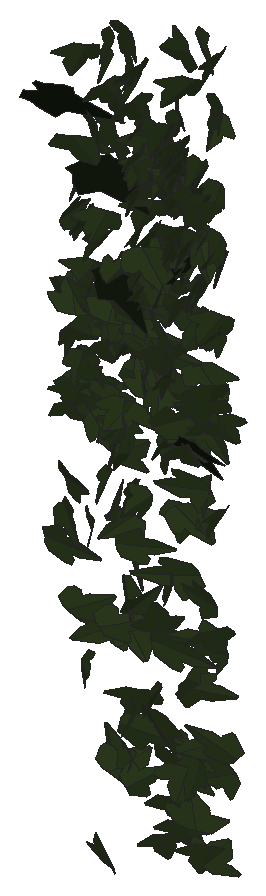
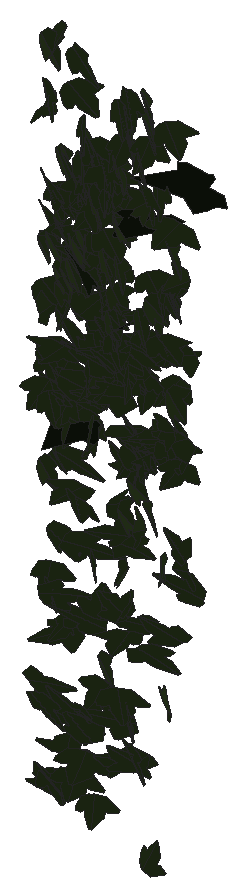
# SketchUp Ruby script. Lengths in millimetres.
U = 1.mm
M = Sketchup.active_model
def pt(a) = Geom::Point3d.new(a.map { |v| v * U })
def face(e, loops, mat)
  f = e.add_face(loops[0].map { |a| pt(a) })
  loops[1..].each { |l| e.add_face(l.map { |a| pt(a) }).erase! }
  f.material = f.back_material = mat if mat
  f
end
# faces: each face lists its corners as indices into pts; further lists are holes
def faces(e, pts, list, mat = nil) = list.each { |f| face(e, (f[0].is_a?(Array) ? f : [f]).map { |l| l.map { |i| pts[i] } }, mat) }
# xy, xz, yz: faces in a plane at the given z, y or x. An outline is a flat list of corners, or four numbers for a rectangle; further outlines are holes
def ring(l) = l.size == 4 ? [[l[0], l[1]], [l[2], l[1]], [l[2], l[3]], [l[0], l[3]]] : l.each_slice(2).to_a
def flat(e, list, mat, &to3) = list.each { |f| face(e, (f[0].is_a?(Array) ? f : [f]).map { |l| ring(l).map { |u, v| to3.(u, v) } }, mat) }
def xy(e, z, list, mat = nil) = flat(e, list, mat) { |x, y| [x, y, z] }
def xz(e, y, list, mat = nil) = flat(e, list, mat) { |x, z| [x, y, z] }
def yz(e, x, list, mat = nil) = flat(e, list, mat) { |y, z| [x, y, z] }
def lines(e, pts, list) = list.each { |a, b| e.add_line(pt(pts[a]), pt(pts[b])) }
# prism: a flat outline (further loops are holes) pulled along v
def prism(e, loops, v, mat = nil)
  f = face(e, loops, mat); d = Geom::Vector3d.new(v.map { |x| x * U })
  f.pushpull(f.normal.samedirection?(d) ? d.length : -d.length)
end
def box(e, o, s, mat = nil) = prism(e, [[o, [o[0] + s[0], o[1], o[2]], [o[0] + s[0], o[1] + s[1], o[2]], [o[0], o[1] + s[1], o[2]]]], [0, 0, s[2]], mat)
def at(x, y, z, deg = 0) = Geom::Transformation.translation(pt([x, y, z])) * Geom::Transformation.rotation(ORIGIN, Z_AXIS, deg.degrees)
def axes(o, x, y, z) = Geom::Transformation.new([*x, 0, *y, 0, *z, 0, *pt(o).to_a, 1])
def part(name) = M.definitions.add(name)
# library, detail: a bought-in or finely detailed component or shape, given as its bounding box
def library(name, o, s) = part(name).tap { |d| box(d.entities, o, s) }
def detail(e, o, s) = box(e.add_group.entities, o, s)
def put(e, d, t, mat = nil) = e.add_instance(d, t).tap { |i| i.material = mat if mat }
def group(e, t, mat = nil) = e.add_group.tap { |g| g.transformation = t; g.material = mat if mat }.entities
root = M.entities
M.materials.add("efeu1").color = [18, 25, 13]
M.materials.add("efeu2").color = [43, 57, 29]
c1 = part("ivyleaf_10")
p = [[0,12.8,-0.8],[-1.5,51.3,-10.9],[-4.9,51,-11.6],[-13.6,26.5,-7.3],[-13.2,15.9,-4.6],[-21.1,19.3,-7.2],
  [-29.5,16.3,-8.3],[-29.2,8.3,-6.2],[-19.7,-9.8,0.5],[-7.6,-13,4],[1,-12.2,5.8],[-0.4,51.1,-11.1],
  [-1.5,51.1,-10.9],[1,-12.4,5.9],[16.9,-12.4,3.5],[35.1,9.1,-5.1],[35,12.9,-6.1],[20.5,16.4,-4.9],
  [15.8,15,-3.8],[15.3,27.6,-7.1],[12.8,31.3,-7.8]]
faces(c1.entities,p,[[0,1,2,3,4,5,6,7,8,9,10],[11,12,0,13,14,15,16,17,18,19,20]],"efeu2")
c2 = part("ivyleaf_9")
p = [[39.1,54.8,31.7],[34.5,51.8,30.2],[-5.3,25.2,17.3],[-17.9,28.3,20.9],[-21.6,21.7,17],[-20.2,4.3,5.3],
  [-22.9,-0.3,2.5],[-17.1,-4,-0.6],[-2,-2.1,-1.2],[-0.7,-15.4,-10.1],[16.6,-22.3,-16.7],[21.1,-15.1,-12.5],
  [32.7,-10.7,-11],[46.1,-1.8,-6.6],[30.8,11.2,3.8]]
faces(c2.entities,p,[[0,1,2,3,4,5,6,7,8,9,10,11,12,13,14]],"efeu1")
put(root,c1,axes([1270.6,1047.9,459],[-0.48285,0.07092,0.58722],[0.98278,-0.28506,0.25752],[0.54901,0.57266,0.05547]))
put(root,c2,axes([1259.8,1017.1,959.8],[0.35127,0.22644,-0.71654],[0.93732,0.52083,0.29145],[1.08021,-0.52557,-0.01989]))
put(root,c1,axes([1290.7,1041.6,666],[0.08143,-0.71118,0.27788],[0.14243,-0.27307,-0.7104],[1.44618,0.06694,0.05432]))
put(root,c1,axes([1286.2,1033.5,567.7],[-0.64923,-0.40429,-0.35378],[0.45804,0.25966,-0.5288],[0.91411,-0.41725,0.01371]))
put(root,c1,axes([1293.5,1040.9,809.3],[0.45294,-0.6195,-0.05972],[-0.02572,0.05878,-0.66359],[1.18422,0.23822,0.00843]))
put(root,c1,axes([1274.2,1035.2,428.7],[0.55128,-0.2534,0.61949],[0.97945,-0.34727,-0.38268],[0.81446,0.58913,0.04089]))
put(root,c1,axes([1299.5,1033.3,593.1],[-0.71097,-0.53152,0.10227],[-0.08643,-0.09305,-0.64947],[1.02652,-0.37597,0.01615]))
put(root,c1,axes([1295.2,1017.3,814.9],[0.19746,-0.12143,0.71883],[-0.29901,0.70528,0.14182],[-1.35485,-0.17335,0.07346]))
put(root,c1,axes([1303.5,1047.5,741.8],[-0.68919,-0.44252,0.31408],[-0.16618,-0.32515,-0.5588],[1.01932,-0.35221,0.12126]))
put(root,c1,axes([1271.1,1024.5,393.3],[-0.1705,-0.0206,0.6802],[1.29073,0.0539,0.09095],[-0.10685,0.68395,0.01332]))
put(root,c1,axes([1299.9,1041.3,809.1],[-0.14305,-0.63344,0.13711],[0.05173,-0.14099,-0.63646],[1.2324,-0.06761,0.04263]))
put(root,c1,axes([1292.6,1037,900.1],[-1.1968,-0.1578,-0.2539],[0.4826,0.03165,-0.64769],[0.30134,-0.67742,0.02889]))
put(root,c1,axes([1284.1,1024.8,721.7],[-0.79131,0.25289,-0.44889],[0.7383,-0.22596,-0.4866],[-0.64532,-0.56861,-0.00627]))
put(root,c1,axes([1300.7,1039.6,807.5],[-0.06985,-0.5542,-0.34902],[0.10152,0.34587,-0.55481],[1.24234,-0.05942,0.02571]))
put(root,c1,axes([1301.3,1017.7,704.4],[0.54287,0.60614,-0.14799],[0.04541,0.152,0.66858],[1.18663,-0.28312,0.04212]))
put(root,c1,axes([1303.2,1029.4,864.3],[0.39037,-0.67223,-0.01479],[0.00033,0.01552,-0.70281],[1.27971,0.20506,0.0047]))
put(root,c1,axes([1307.4,1027.7,1026.5],[-0.56433,-0.63131,0.13286],[-0.04648,-0.13513,-0.69661],[1.22695,-0.29549,0.03472]))
put(root,c1,axes([1291.5,1051,624.8],[-0.50661,0.32371,-0.48857],[0.53245,-0.40133,-0.41833],[-0.98013,-0.38534,0.02527]))
put(root,c1,axes([1298.9,1022.8,673.5],[-0.4007,-0.39208,-0.52059],[0.46515,0.45965,-0.44503],[1.14983,-0.32258,-0.00138]))
put(root,c1,axes([1295,1047.7,236.8],[-0.08005,-0.11947,-0.66552],[0.28496,-0.65189,0.10756],[-1.25491,-0.14041,0.06688]))
put(root,c1,axes([1299.5,1029.8,632.5],[0.81136,-0.41907,0.26503],[0.33228,-0.20028,-0.5975],[0.88325,0.4603,-0.01868]))
put(root,c1,axes([1290.9,1031.7,601.4],[-0.59807,-0.21352,-0.5687],[0.98704,0.23908,-0.37634],[0.60197,-0.60416,0.05206]))
put(root,c1,axes([1314.7,1030.7,423.7],[0.18319,-0.2164,-0.62084],[-0.10033,0.6229,-0.22529],[1.24728,0.08189,0.07306]))
put(root,c1,axes([1320.1,1045.9,787.2],[0.01443,-0.57265,0.3385],[0.01646,-0.3384,-0.57269],[1.26592,0.01093,0.00359]))
put(root,c1,axes([1302.7,1034.1,604.2],[0.18724,0.03395,0.63404],[0.5869,0.55831,-0.07774],[-1.05635,0.3162,0.06919]))
put(root,c1,axes([1316.3,1036,745.6],[0.49908,-0.57185,0.15686],[0.16781,-0.132,-0.62863],[1.11599,0.27558,0.02438]))
put(root,c1,axes([1333.4,1041.6,299.4],[0.86718,0.14801,-0.46596],[-0.84348,-0.14387,-0.47908],[-0.39283,0.63563,0.00007]))
put(root,c1,axes([1301.9,1024.3,321.7],[0.70088,0.10938,-0.51488],[0.94066,0.14429,0.38416],[0.34459,-0.61636,-0.00144]))
put(root,c1,axes([1324.7,1024.3,937.2],[0.74216,-0.4563,-0.37185],[-0.02289,0.43978,-0.55226],[1.12004,0.31134,0.23511]))
put(root,c1,axes([1328.1,1037.8,817.7],[-0.67576,-0.50671,0.22798],[0.00591,-0.27236,-0.60051],[1.05748,-0.32228,0.14905]))
put(root,c1,axes([1332.1,1038.9,3.3],[-0.90347,0.42743,-0.05893],[-0.08592,0.03792,0.63878],[0.81667,0.47685,0.00202]))
put(root,c1,axes([1335.7,1038.1,933.8],[0.78445,-0.49191,-0.26423],[-0.13252,0.28057,-0.63096],[1.05442,0.40123,0.11728]))
put(root,c1,axes([1327.7,1027.1,564.8],[0.22158,0.70117,0.19962],[0.06315,0.19685,-0.71077],[-1.38606,0.12106,-0.00047]))
put(root,c1,axes([1313,1038.7,590.9],[-0.53445,0.01322,-0.60596],[1.11303,-0.16953,-0.27472],[-0.30303,-0.646,0.05969]))
put(root,c1,axes([1333.1,1036.7,492.4],[0.54302,-0.59955,0.11204],[0.12132,-0.0937,-0.66376],[1.15445,0.29185,0.01705]))
put(root,c1,axes([1337.1,1033,662.6],[-0.46875,-0.56282,-0.21689],[0.1793,0.19551,-0.61431],[1.13386,-0.26359,0.00747]))
put(root,c1,axes([1340,1042.7,762.2],[-0.02894,-0.64209,-0.11858],[0.02389,0.11831,-0.6422],[1.24247,-0.01723,0.00959]))
put(root,c1,axes([1342,1028.2,1025],[0.4556,-0.66517,-0.10263],[-0.02225,0.10481,-0.70652],[1.28073,0.23844,0.02423]))
put(root,c1,axes([1348.5,1037,139.2],[0.92508,-0.27392,0.41375],[-0.68435,0.20469,0.55794],[-0.65079,-0.60461,0.00143]))
put(root,c1,axes([1355.8,1029.8,976.4],[-0.40267,0.41784,0.51326],[-0.80618,0.32854,-0.44207],[-0.96783,-0.44751,0.15469]))
put(root,c1,axes([1328.5,1039.1,679.8],[0.92068,-0.23299,0.34543],[0.6499,-0.08161,-0.53325],[0.4544,0.5888,0.06278]))
put(root,c1,axes([1341.2,1025.6,991.9],[-0.51206,-0.54368,-0.37865],[0.32502,0.33796,-0.60661],[1.21834,-0.31866,0.00268]))
put(root,c1,axes([1349.8,1030.1,457.8],[0.27821,-0.30767,0.66519],[-0.57251,0.59334,0.34054],[-1.27194,-0.33436,-0.00778]))
put(root,c1,axes([1347.6,1023.2,1052.2],[0.49675,-0.66081,-0.1576],[-0.04579,0.15973,-0.70961],[1.29212,0.25971,0.03544]))
put(root,c1,axes([1344.2,1051.1,532.2],[0.27646,-0.54386,0.4039],[0.18386,-0.39222,-0.56288],[1.27611,0.17433,-0.0064]))
put(root,c1,axes([1319.7,1031.1,713.1],[-0.02383,-0.01891,0.72738],[1.38011,-0.0603,0.01092],[0.11416,0.72499,0.01988]))
put(root,c1,axes([1347,1038.5,541.5],[0.18033,-0.49313,-0.41549],[0.15147,0.42569,-0.48708],[1.21787,0.02008,0.1221]))
put(root,c1,axes([1357.9,1037.8,567.6],[-0.40893,-0.47748,0.38443],[-0.28507,-0.35412,-0.52355],[1.13131,-0.26182,0.00703]))
put(root,c1,axes([1340.2,1039.8,918.9],[-0.69761,0.44971,-0.37639],[0.40815,-0.31033,-0.57963],[-1.03881,-0.42393,0.02503]))
put(root,c1,axes([1357.1,1046.1,440.6],[0.52032,0.33514,-0.47041],[-0.63122,-0.335,-0.43142],[-0.89996,0.42872,0.03062]))
put(root,c1,axes([1360.2,1035.4,146.4],[0.39469,-0.40776,-0.52662],[-0.45604,0.46895,-0.45747],[1.18272,0.3169,-0.00065]))
put(root,c1,axes([1347.8,1024.9,754.1],[0.12771,0.21097,-0.64366],[0.39072,0.61005,0.22136],[1.2285,-0.21596,-0.00349]))
put(root,c2,axes([1338.3,1018.8,891.4],[-0.11232,-0.38165,-0.68878],[0.28644,0.67252,-0.38553],[1.47105,-0.16009,0.02248]))
put(root,c1,axes([1348.4,1023.2,708.4],[0.66981,0.50858,-0.26519],[0.29588,0.2149,0.61845],[1.05074,-0.38471,-0.0051]))
put(root,c1,axes([1354,1033.9,567.3],[0.72092,-0.5372,0.01208],[0.00676,-0.01227,-0.65731],[1.02264,0.37879,-0.00417]))
put(root,c1,axes([1338,1042.6,586],[0.39302,-0.37848,-0.50768],[0.63464,-0.38896,0.42561],[-1.02453,-0.38612,0.06889]))
put(root,c1,axes([1360.5,1033.7,701.1],[1.25707,-0.26821,-0.18791],[-0.33272,0.06893,-0.71288],[0.52704,0.68324,-0.00184]))
put(root,c1,axes([1361.4,1036.5,671.1],[-0.01576,-0.5128,-0.43211],[0.06005,0.43136,-0.51252],[1.27484,-0.02666,0.0188]))
put(root,c1,axes([1361,1037.6,1057.8],[0.88218,-0.44354,-0.28824],[-0.0789,0.35161,-0.60772],[1.00364,0.4175,0.20558]))
put(root,c1,axes([1365.8,1033.2,591.6],[1.05492,0.251,-0.26853],[-0.46171,-0.11522,-0.60845],[-0.52557,0.60504,-0.00446]))
put(root,c1,axes([1368.7,1034.6,205.4],[0.3316,-0.57237,-0.44109],[-0.22403,0.42519,-0.59823],[1.3569,0.21008,0.00903]))
put(root,c1,axes([1357.6,1043.8,359.4],[-0.14189,0.65091,-0.32371],[0.05772,-0.32234,-0.65514],[-1.38235,-0.08027,0.00587]))
put(root,c1,axes([1385.2,1039.1,692.2],[0.48163,0.09367,-0.64986],[-1.24953,0.04326,-0.24943],[0.01284,0.69605,0.10296]))
put(root,c1,axes([1364.3,1032.7,707.6],[1.25656,-0.31949,-0.08331],[-0.14244,0.03659,-0.73348],[0.61203,0.66447,0.00033]))
put(root,c1,axes([1351,1034.9,569.8],[1.06192,-0.14282,0.29236],[0.5543,-0.03953,-0.57516],[0.27609,0.62868,0.03025]))
put(root,c2,axes([1350.5,1029.4,752.4],[0.32907,-0.73216,-0.23493],[-0.0675,0.23295,-0.75208],[1.46186,0.17557,0.01816]))
put(root,c1,axes([1361.9,1048.4,483.4],[0.32525,-0.54536,0.41093],[0.27289,-0.3855,-0.57124],[1.27062,0.22239,0.0175]))
put(root,c1,axes([1372.2,1045.6,226.1],[-0.94768,-0.43541,0.05291],[-0.07469,-0.0355,-0.66145],[0.83141,-0.49948,0.00089]))
put(root,c1,axes([1351.6,1033.2,131.9],[0.88201,0.20908,-0.50218],[0.76017,0.31707,0.50061],[0.70282,-0.60533,0.08876]))
put(root,c1,axes([1371.5,1028.7,1024.6],[0.36167,-0.57376,-0.38438],[-0.10155,0.38528,-0.60148],[1.31045,0.18821,0.05947]))
put(root,c1,axes([1351.5,1019.2,318.6],[0.41869,0.06257,-0.60972],[0.93689,0.36791,0.21537],[0.69499,-0.53367,0.07699]))
put(root,c1,axes([1393,1035.7,672.5],[-0.45318,0.01834,0.63],[-1.19951,-0.00386,-0.2381],[-0.00547,-0.67348,0.01852]))
put(root,c1,axes([1377.3,1025.1,1005.5],[0.36185,-0.65849,-0.24032],[-0.13364,0.22986,-0.68538],[1.32738,0.20265,-0.00349]))
put(root,c1,axes([1376.3,1044,716.6],[-0.43925,-0.59385,-0.05254],[0.02259,0.05175,-0.63708],[1.13441,-0.23097,-0.00765]))
put(root,c1,axes([1371,1017.2,544.3],[-0.1275,-0.29486,-0.60653],[0.27566,0.589,-0.30234],[1.25357,-0.15951,0.0048]))
put(root,c1,axes([1368.4,1040,399.6],[-0.38242,0.57916,-0.17977],[0.11339,-0.16961,-0.61302],[-1.14855,-0.20958,-0.00067]))
put(root,c1,axes([1366.8,1038.9,308.6],[0.69472,0.54256,0.17209],[0.16991,0.14733,-0.65387],[-1.06989,0.3757,0.0079]))
put(root,c1,axes([1378.4,1037.2,819.4],[0.13486,-0.64045,-0.17021],[0.01214,0.17183,-0.6439],[1.26116,0.06683,0.0244]))
put(root,c1,axes([1360.4,1029.7,535.2],[0.89029,-0.20882,-0.40512],[0.70093,-0.16879,0.51227],[-0.51098,-0.59536,-0.00314]))
put(root,c1,axes([1384.1,1031.6,957.4],[0.15377,-0.66352,-0.23934],[-0.09301,0.23506,-0.66816],[1.33924,0.09251,-0.01892]))
put(root,c1,axes([1379,1027.1,982.3],[-0.44774,-0.54082,-0.40317],[0.30141,0.37077,-0.58977],[1.24794,-0.28359,-0.00221]))
put(root,c1,axes([1374.5,1037.1,338.1],[-0.22071,-0.56844,0.34966],[0.12959,0.34297,0.58014],[-1.26352,0.13447,-0.00158]))
put(root,c1,axes([1384.4,1026.6,1029.8],[-0.19237,-0.67884,-0.18934],[0.01258,0.19036,-0.68601],[1.34122,-0.09915,-0.02072]))
put(root,c1,axes([1384.8,1043.3,744.8],[-0.01025,-0.64528,-0.01357],[0.00213,0.01356,-0.6453],[1.22836,-0.00541,0.00101]))
put(root,c1,axes([1385.3,1035.4,777],[-0.12923,-0.63604,0.13574],[0.01058,-0.13704,-0.63935],[1.23772,-0.06524,0.01964]))
put(root,c1,axes([1383.3,1032.1,874.6],[0.24769,-0.63696,0.17304],[0.07285,-0.16879,-0.65011],[1.25409,0.13561,0.00359]))
put(root,c1,axes([1396.8,1030.4,743.2],[0.8845,-0.12951,0.46006],[-0.84324,0.12388,0.48245],[-0.34109,-0.6421,0.00029]))
put(root,c1,axes([1386.6,1036.3,481.7],[-0.21206,-0.12033,0.64185],[0.2085,-0.64535,-0.10197],[1.22525,0.08899,0.12844]))
put(root,c1,axes([1387,1027.6,922.1],[-0.22058,-0.54203,-0.39898],[0.21664,0.38324,-0.55371],[1.26249,-0.16047,0.02531]))
put(root,c1,axes([1393.9,1040.2,854],[-0.62893,-0.55119,0.19166],[-0.08677,-0.19519,-0.63997],[1.10723,-0.32838,0.05871]))
put(root,c1,axes([1402.8,1040,736.2],[-0.89109,0.21017,0.39693],[-0.73252,0.10775,-0.51106],[-0.44055,-0.60428,0.04692]))
put(root,c1,axes([1392.3,1034.2,910.6],[-0.35435,-0.6015,0.31164],[0.00541,-0.32389,-0.62344],[1.28928,-0.16396,0.08827]))
put(root,c1,axes([1379.2,1026,124.8],[0.25153,0.20273,-0.6363],[0.65435,0.53541,0.242],[1.08959,-0.36834,0.00156]))
put(root,c1,axes([1396.6,1030.8,627.3],[0.36142,0.66022,-0.04458],[-0.0353,0.05168,0.68624],[1.25889,-0.18809,0.03204]))
put(root,c1,axes([1397.8,1035.9,938.9],[-0.98352,-0.47524,0.07532],[0.0776,-0.15338,-0.68803],[0.91247,-0.4992,0.13969]))
put(root,c1,axes([1399.3,1036.9,823.5],[0.01964,-0.6808,-0.11343],[-0.03246,0.11316,-0.68071],[1.31315,0.01298,-0.01513]))
put(root,c1,axes([1401.8,1043.1,731.4],[0.90978,-0.41019,-0.22241],[-0.31775,0.14696,-0.62989],[0.82925,0.50634,0.00265]))
put(root,c1,axes([1371.1,1037.8,187.1],[-0.18733,-0.04671,-0.70152],[1.33785,0.00683,-0.09909],[0.02525,-0.70836,0.0453]))
put(root,c1,axes([1400.6,1028.9,905.5],[0.45807,-0.62018,-0.23706],[-0.09905,0.23376,-0.66438],[1.25973,0.24389,0.03397]))
put(root,c1,axes([1391.5,1029.6,636.3],[-0.23697,0.50445,-0.38803],[0.1378,-0.38159,-0.51931],[-1.20337,-0.14303,0.01694]))
put(root,c1,axes([1400.4,1025.7,665],[0.46411,-0.55145,-0.29118],[-0.07166,0.29906,-0.59791],[1.18467,0.23413,0.07791]))
put(root,c1,axes([1374.8,1038.9,637.5],[-0.33638,-0.09364,-0.70528],[1.32248,0.13336,-0.19184],[0.29082,-0.71476,0.0566]))
put(root,c1,axes([1382.8,1014.2,431.1],[-0.07345,-0.02389,0.66397],[0.68263,0.5591,0.04096],[-1.06439,0.36022,-0.01955]))
put(root,c1,axes([1399.1,1037.9,950.3],[0.98762,-0.45673,-0.11867],[-0.00527,0.17343,-0.67962],[0.8981,0.50328,0.12651]))
put(root,c1,axes([1380.2,1028.6,691.6],[-0.03396,-0.10358,-0.65219],[1.11184,0.30172,-0.0639],[0.58598,-0.57848,0.08345]))
put(root,c1,axes([1401.7,1034.5,919.7],[0.44498,-0.5929,-0.29713],[0.06832,0.32591,-0.62207],[1.26033,0.19166,0.13863]))
put(root,c1,axes([1406.8,1037.5,912.6],[-0.23053,-0.62782,0.29259],[-0.05532,-0.29216,-0.63893],[1.3171,-0.12216,0.02437]))
put(root,c1,axes([1406.3,1038.5,328.5],[-0.74392,-0.5114,-0.17382],[-0.20667,-0.13577,0.64367],[-1.007,0.40566,-0.0037]))
put(root,c1,axes([1408.7,1042.2,895.6],[-1.10953,-0.36605,-0.00176],[-0.00616,0.00847,-0.68832],[0.69665,-0.58292,-0.00889]))
put(root,c1,axes([1397.9,1028.2,905.9],[-0.90971,-0.28981,-0.39055],[0.6792,0.16301,-0.55773],[0.6288,-0.59534,0.03741]))
put(root,c1,axes([1410.8,1026.6,249.9],[0.36047,-0.64026,0.08217],[0.03707,-0.07993,-0.66767],[1.22798,0.19036,-0.00397]))
put(root,c1,axes([1413.1,1041.9,902],[0.15443,-0.66509,-0.15393],[-0.04096,0.15245,-0.67002],[1.29862,0.0839,-0.00283]))
put(root,c1,axes([1420.4,1050.9,748.1],[-0.47319,-0.32018,-0.50653],[-0.61281,-0.39112,0.40527],[-0.96184,0.40671,-0.00902]))
put(root,c1,axes([1413.9,1040.1,61.7],[-0.62093,-0.54441,-0.12974],[0.15005,0.10397,-0.63453],[1.05451,-0.33536,0.01389]))
put(root,c1,axes([1407.8,1031,216.4],[-1.13269,0.42501,-0.17549],[0.27098,-0.10259,-0.73133],[-0.83211,-0.61194,0.00072]))
put(root,c1,axes([1415.4,1031.3,810.8],[0.81829,-0.46886,-0.18478],[-0.06046,0.21719,-0.62502],[0.95723,0.41453,0.11848]))
put(root,c1,axes([1402.2,1021.2,799.2],[1.11846,0.37901,0.26824],[0.41596,0.15596,-0.69919],[-0.7797,0.62689,0.01177]))
put(root,c1,axes([1417.7,1025.4,764.3],[0.377,-0.62649,-0.21894],[0.0227,0.23181,-0.65252],[1.26285,0.18286,0.07709]))
put(root,c1,axes([1421.1,1031.4,963.5],[-0.39116,-0.66648,0.16178],[-0.03145,-0.16403,-0.69673],[1.3049,-0.20374,0.0317]))
put(root,c1,axes([1410.7,1037.1,887.7],[-0.71979,-0.44886,-0.43311],[0.56903,0.31407,-0.58657],[1.04185,-0.48164,0.02114]))
put(root,c1,axes([1434.7,1034.1,741.3],[0.64133,-0.01814,-0.55069],[-0.99192,0.19893,-0.32547],[0.3402,0.6142,0.08915]))
put(root,c1,axes([1415.9,1028.1,626.4],[0.41746,0.60907,-0.19533],[-0.15031,-0.17912,-0.64723],[-1.20802,0.23277,0.01303]))
put(root,c1,axes([1435,1016.9,703.5],[-0.27589,0.25713,-0.65999],[-0.61824,0.57452,0.29518],[1.19794,0.35572,0.00034]))
put(root,c1,axes([1419.4,1032.6,652.2],[0.16407,-0.4078,-0.61317],[0.2216,0.61714,-0.39407],[1.38388,-0.05047,0.1358]))
put(root,c1,axes([1426,1022.7,688.6],[-0.72233,-0.60035,-0.04],[0.03191,0.03673,-0.71024],[1.14468,-0.37987,-0.00545]))
put(root,c1,axes([1422.1,1035.6,910.2],[-0.19242,-0.51814,0.45118],[0.17859,-0.46218,-0.50974],[1.29533,-0.01325,0.1373]))
put(root,c1,axes([1424.2,1031.6,656],[-0.11587,-0.50013,-0.40046],[0.05615,0.39965,-0.5036],[1.21809,-0.066,-0.01488]))
put(root,c1,axes([1423.8,1023.6,558.3],[0.21452,-0.15889,-0.69018],[0.1458,0.6975,-0.14806],[1.34,-0.05045,0.1266]))
put(root,c1,axes([1425.3,1022.9,575],[-0.07127,-0.42888,-0.50986],[0.10696,0.50681,-0.43044],[1.26349,-0.06709,0.00768]))
put(root,c1,axes([1426.6,1036,904.7],[-0.22227,-0.67361,0.04651],[0.12583,-0.05838,-0.67954],[1.2789,-0.11133,0.07494]))
put(root,c1,axes([1447.6,1034.8,406.9],[0.37946,0.06023,-0.72349],[-1.30509,-0.23076,-0.20819],[-0.45373,0.71411,-0.00625]))
put(root,c1,axes([1430.3,1017.6,892.7],[-1.0117,0.39674,0.17608],[-0.24275,0.12334,-0.66295],[-0.78964,-0.54623,-0.0218]))
put(root,c1,axes([1436,1035.5,994.3],[-0.45788,0.46905,0.46053],[-0.61734,0.34183,-0.51761],[-1.08813,-0.39131,0.09987]))
put(root,c1,axes([1400.6,1039.7,670],[0.31911,-0.1235,-0.67754],[1.22819,-0.21538,0.19896],[-0.45779,-0.66391,0.06149]))
put(root,c1,axes([1423,1040.6,913.7],[-1.02553,-0.3769,-0.19542],[0.42654,0.01565,-0.64817],[0.68624,-0.57297,0.11084]))
put(root,c1,axes([1431.5,1024.4,394.1],[0.41889,-0.54576,-0.24506],[-0.05991,0.25019,-0.58547],[1.13702,0.21425,0.05943]))
put(root,c1,axes([1452.9,1040.5,632.3],[-0.22213,-0.04175,0.64948],[-1.20397,-0.14775,-0.12318],[0.29102,-0.64313,-0.01386]))
put(root,c1,axes([1432.5,1032.2,933],[-0.09263,-0.69172,0.02561],[-0.00297,-0.02556,-0.69343],[1.31738,-0.0487,0.00024]))
put(root,c1,axes([1432.6,1038.8,944.4],[-0.20264,-0.68909,-0.0452],[0.02229,0.04392,-0.69725],[1.3141,-0.107,0.00486]))
put(root,c1,axes([1433.8,1039.6,917.6],[-0.35714,0.64918,0.15496],[-0.37453,0.09999,-0.65722],[-1.21376,-0.22187,0.1572]))
put(root,c1,axes([1430.4,1037.5,935],[0.15897,-0.67056,-0.16265],[0.12429,0.17078,-0.67056],[1.30732,0.0653,0.08353]))
put(root,c1,axes([1432.2,1032.5,974.3],[0.55106,-0.64363,-0.11627],[-0.00659,0.12565,-0.70414],[1.24477,0.2856,0.04775]))
put(root,c1,axes([1433.4,1037.2,114.2],[-1.13658,-0.31465,-0.15769],[0.26453,0.07448,-0.67501],[0.61538,-0.61315,-0.00107]))
put(root,c2,axes([1446.2,1025.5,794.6],[-0.08474,0.53285,0.54734],[-0.05117,0.54684,-0.53455],[-1.45292,-0.05034,-0.0131]))
put(root,c1,axes([1436.5,1042.8,827.8],[0.19516,-0.60463,0.26286],[0.05302,-0.26181,-0.61308],[1.25366,0.1052,-0.01499]))
put(root,c1,axes([1455.9,1023.3,1076.9],[-0.53288,0.21572,0.6234],[-1.12007,0.22425,-0.34193],[-0.56716,-0.64555,0.08954]))
put(root,c1,axes([1421.1,1045.6,154.9],[-0.8903,-0.05026,0.4431],[0.844,0.01509,0.46989],[-0.08924,0.64415,0.02356]))
put(root,c1,axes([1425.2,1038.9,814.3],[1.10782,0.24251,0.22579],[0.39096,0.09401,-0.63054],[-0.49481,0.61722,0.00732]))
put(root,c1,axes([1438.1,1023.6,826.1],[0.13159,-0.58898,-0.31305],[0.12554,0.31922,-0.58602],[1.26322,0.02963,0.09085]))
put(root,c1,axes([1440.4,1034.3,919.9],[0.15015,-0.68053,0.16412],[0.03461,-0.16311,-0.68509],[1.33187,0.08096,-0.0007]))
put(root,c1,axes([1431.9,1047.8,476.1],[1.10763,-0.29155,0.13847],[0.2339,-0.06383,-0.65092],[0.56801,0.59481,-0.00198]))
put(root,c1,axes([1440.1,1031.1,840.2],[0.18439,-0.61001,0.28124],[0.05952,-0.27975,-0.61754],[1.27703,0.10112,-0.01182]))
put(root,c1,axes([1435.4,1034.4,835.9],[-1.26502,-0.01113,-0.20775],[0.39489,0.01547,-0.66468],[0.02899,-0.69622,-0.01144]))
put(root,c1,axes([1444.1,1036.7,752.4],[0.02457,-0.63852,0.17564],[-0.02655,-0.1759,-0.63843],[1.26009,0.00874,-0.01688]))
put(root,c1,axes([1442.6,1039.4,86.8],[-1.02287,-0.34916,-0.13508],[0.21064,0.07759,-0.64089],[0.68066,-0.5487,-0.00466]))
put(root,c1,axes([1452.3,1029.7,1032.8],[-0.4707,-0.58792,0.33025],[-0.25704,-0.30145,-0.63779],[1.25737,-0.28171,-0.00675]))
put(root,c1,axes([1445.9,1044.5,796],[0.14895,-0.65679,0.00898],[0.00142,-0.00896,-0.66144],[1.25012,0.07827,-0.00032]))
put(root,c1,axes([1432.4,1018.6,598.4],[-0.25508,-0.33783,0.67271],[0.44238,0.63133,0.36336],[-1.36268,0.26819,-0.00796]))
put(root,c1,axes([1416.7,1034.8,307],[-0.05065,0.0114,0.75508],[1.41001,0.14678,0.02389],[-0.27845,0.74116,-0.01635]))
put(root,c1,axes([1465.4,1034.1,522.7],[0.5418,-0.08203,-0.61214],[-1.12045,0.1677,-0.29626],[0.3553,0.65393,-0.00081]))
put(root,c1,axes([1447,1024.8,935.4],[-0.05335,-0.5891,-0.3551],[0.09285,0.3528,-0.58913],[1.30582,-0.04915,0.02738]))
put(root,c1,axes([1448.9,1035.9,826],[0.29257,-0.66291,0.10212],[0.03769,-0.10024,-0.6805],[1.27598,0.15496,-0.00332]))
put(root,c1,axes([1455.4,1033.4,893.4],[-0.26934,-0.64937,0.18779],[-0.06327,-0.18494,-0.66458],[1.28496,-0.14522,0.00664]))
put(root,c1,axes([1449,1029.3,157.4],[1.25852,0.04672,-0.04449],[-0.08536,0.00365,-0.66288],[-0.08825,0.66275,0.00678]))
put(root,c1,axes([1454.2,1045.2,716.9],[0.96173,-0.40252,-0.09325],[-0.12429,0.06764,-0.64593],[0.77647,0.50938,0.01209]))
put(root,c1,axes([1454.8,1053.4,767.9],[0.00623,-0.49757,0.40547],[0.14514,-0.4023,-0.4943],[1.21293,0.05069,0.05707]))
put(root,c1,axes([1454.2,1029.5,573.3],[-0.51617,-0.5559,-0.2919],[0.25224,0.26012,-0.61851],[1.16805,-0.30183,0.00458]))
put(root,c2,axes([1444.7,1028.4,578.4],[1.41827,0.01057,-0.14491],[-0.27609,0.01144,-0.74516],[-0.01558,0.75908,0.01325]))
put(root,c1,axes([1455.4,1041.6,733.5],[-0.41425,0.6227,0.01951],[-0.0169,0.01756,-0.65964],[-1.18558,-0.21783,0.00259]))
put(root,c1,axes([1438.8,1042.9,177.3],[0.92363,-0.1457,-0.42236],[0.80784,-0.04429,0.503],[-0.26542,-0.64183,0.06117]))
put(root,c1,axes([1442.4,1034.1,592.4],[1.0356,0.22993,0.3502],[0.59212,0.16265,-0.5902],[-0.53396,0.62631,0.02471]))
put(root,c1,axes([1445.1,1034,483.6],[0.64916,0.43905,0.38721],[0.46481,0.30056,-0.55593],[-1.01255,0.41945,-0.00695]))
put(root,c1,axes([1460.3,1039.3,599.7],[-1.06734,0.34214,-0.00262],[0.00307,-0.00238,-0.65694],[-0.65116,-0.56081,0.00119]))
put(root,c1,axes([1458.7,1040,779.9],[0.42424,-0.54803,0.2909],[0.17757,-0.27598,-0.59141],[1.1674,0.24113,-0.01575]))
put(root,c1,axes([1478.3,1044.1,328.8],[0.05421,0.09722,0.66532],[-0.70894,-0.55211,0.09662],[1.06536,-0.37234,0.03044]))
put(root,c1,axes([1485.8,1028.3,619.4],[-0.1525,0.00077,0.65378],[-1.23922,0.05918,-0.07987],[-0.11197,-0.656,-0.00643]))
put(root,c1,axes([1467.3,1036.2,886.9],[-0.24375,-0.65332,0.20822],[0.00229,-0.21203,-0.66455],[1.30501,-0.12165,0.04006]))
put(root,c1,axes([1464.6,1029.8,931.4],[0.68928,-0.57965,0.04082],[0.02985,-0.03833,-0.68345],[1.10551,0.36244,-0.00699]))
put(root,c1,axes([1459.2,1050.5,732.1],[0.1461,-0.47822,0.43051],[0.40324,-0.3906,-0.47166],[1.15633,0.19663,0.11009]))
put(root,c1,axes([1467.4,1041.6,779.7],[0.33344,-0.61482,0.26618],[0.13775,-0.25615,-0.6393],[1.26762,0.18956,-0.00055]))
put(root,c1,axes([1471.8,1025,884.6],[-0.79759,-0.54577,-0.09012],[0.08375,0.07981,-0.68797],[1.04944,-0.42116,-0.01359]))
put(root,c1,axes([1468,1024.9,107.1],[1.18654,0.24269,0.04127],[-0.09108,0.00925,0.66851],[0.45959,-0.62474,0.02593]))
put(root,c1,axes([1465.2,1028.6,171.9],[1.00636,-0.48718,0.12363],[0.17895,-0.08039,-0.71897],[0.9397,0.53705,0.00452]))
put(root,c1,axes([1470.1,1037.9,844.4],[0.49921,-0.63727,0.14417],[0.08466,-0.13757,-0.68905],[1.24061,0.26582,-0.01099]))
put(root,c1,axes([1465.5,1020.3,287.7],[-0.28312,-0.39023,-0.5446],[0.46728,0.4873,-0.41624],[1.1864,-0.28506,0.03398]))
put(root,c1,axes([1476,1026.6,931.8],[0.28895,-0.69872,-0.00348],[0.00444,0.00407,-0.71502],[1.32981,0.15181,0.00314]))
put(root,c1,axes([1477.7,1045.3,601.5],[-0.43538,-0.6235,-0.0101],[0.00859,0.0091,-0.66414],[1.18677,-0.22881,0.00111]))
put(root,c1,axes([1480.3,1031.8,71.3],[-0.84331,-0.48512,0.07064],[-0.09008,-0.05245,-0.65703],[0.92867,-0.44562,0.00042]))
put(root,c1,axes([1493.3,1016,396.7],[0.1624,-0.0376,-0.63001],[-0.84462,0.44846,-0.08687],[0.85407,0.45064,0.03389]))
put(root,c1,axes([1464.8,1024.9,275.6],[-0.37117,-0.19922,-0.6954],[0.9528,0.48271,-0.27869],[0.99375,-0.53722,0.00747]))
put(root,c1,axes([1470.6,1042.2,528],[0.59661,-0.42078,0.45178],[0.52411,-0.35818,-0.52468],[1.05162,0.41722,0.00519]))
put(root,c1,axes([1499.8,1042,198.3],[0.5146,0.0986,0.58055],[-1.09034,-0.10371,0.28443],[0.25922,-0.63198,0.0439]))
put(root,c1,axes([1481.5,1038.6,819.7],[0.31631,-0.64425,0.18527],[0.08367,-0.17999,-0.66534],[1.27308,0.1719,-0.00231]))
put(root,c1,axes([1480.2,1021.3,1100.3],[-0.49028,0.67358,0.02736],[-0.03479,0.0223,-0.7211],[-1.28254,-0.2581,0.0091]))
put(root,c1,axes([1478.4,1025,832.8],[0.27221,0.66193,-0.02644],[-0.01094,-0.02581,-0.67721],[-1.26074,0.14314,0.00017]))
put(root,c1,axes([1469.3,1037.5,671],[1.00498,0.24001,0.31496],[0.53972,0.1372,-0.58],[-0.52601,0.59934,0.00665]))
put(root,c1,axes([1489.6,1023.3,641.6],[-0.76313,-0.54568,-0.01251],[0.01891,0.00822,-0.67715],[1.03864,-0.40108,0.00314]))
put(root,c1,axes([1482.3,1043.7,901.5],[0.9002,-0.49863,0.15825],[0.2099,-0.11351,-0.68728],[0.97327,0.48568,0.00185]))
put(root,c1,axes([1492.1,1024.4,661.6],[-0.57505,-0.6049,0.05545],[-0.04201,-0.05096,-0.67616],[1.15531,-0.30294,0.00301]))
put(root,c1,axes([1494.2,1031.8,747.2],[-0.5656,-0.49884,0.3104],[-0.10461,-0.32272,-0.57126],[1.11327,-0.28376,0.10402]))
put(root,c1,axes([1490.3,1045.3,721.1],[-0.10911,0.00792,-0.69212],[-0.32367,-0.67336,0.00639],[-1.27695,0.17,0.05752]))
put(root,c1,axes([1501.4,1038.1,172.8],[0.79167,-0.30166,-0.43247],[-0.66295,0.25632,-0.51383],[0.75338,0.54255,0.0023]))
put(root,c1,axes([1475.2,1036.9,56.4],[1.13886,-0.1076,-0.28282],[0.53921,-0.02091,0.6074],[-0.20229,-0.66153,0.02681]))
put(root,c1,axes([1501.1,1029.8,330.1],[0.35689,-0.34002,-0.50703],[-0.46987,0.44287,-0.3883],[1.06264,0.31002,-0.0014]))
put(root,c1,axes([1487.3,1049.4,815.8],[0.44943,-0.53655,0.27118],[0.24932,-0.23842,-0.58582],[1.11668,0.26918,0.02165]))
put(root,c1,axes([1493.6,1037.9,500.2],[0.03782,-0.63703,0.16866],[0.01847,-0.16843,-0.63732],[1.25403,0.02169,0.0043]))
put(root,c1,axes([1488.6,1039.2,613.6],[-0.85415,-0.41114,-0.31279],[0.42225,0.22078,-0.60854],[0.88789,-0.50051,-0.0115]))
put(root,c1,axes([1471,1037.2,604.8],[0.85743,-0.16717,0.56701],[1.03933,-0.15526,-0.47968],[0.43076,0.70736,0.02871]))
put(root,c1,axes([1493.2,1025.9,352.1],[-0.65035,-0.53042,-0.18311],[0.2012,0.14969,-0.63092],[1.04883,-0.35761,0.00749]))
put(root,c1,axes([1495.5,1029.2,847.2],[0.84559,-0.50245,-0.0583],[-0.06837,0.04605,-0.6707],[0.96025,0.44573,0.00358]))
put(root,c1,axes([1498,1027.4,1084.4],[0.09145,-0.71284,0.10847],[-0.01768,-0.10932,-0.71427],[1.37219,0.0461,-0.01643]))
put(root,c1,axes([1494.2,1034.8,999.4],[0.1882,0.49572,-0.49573],[-0.18306,-0.48631,-0.50549],[-1.32165,0.13795,-0.00058]))
put(root,c1,axes([1499.2,1025.4,1018],[0.64463,-0.54812,-0.3443],[-0.1064,0.36236,-0.63188],[1.22731,0.31931,0.12606]))
